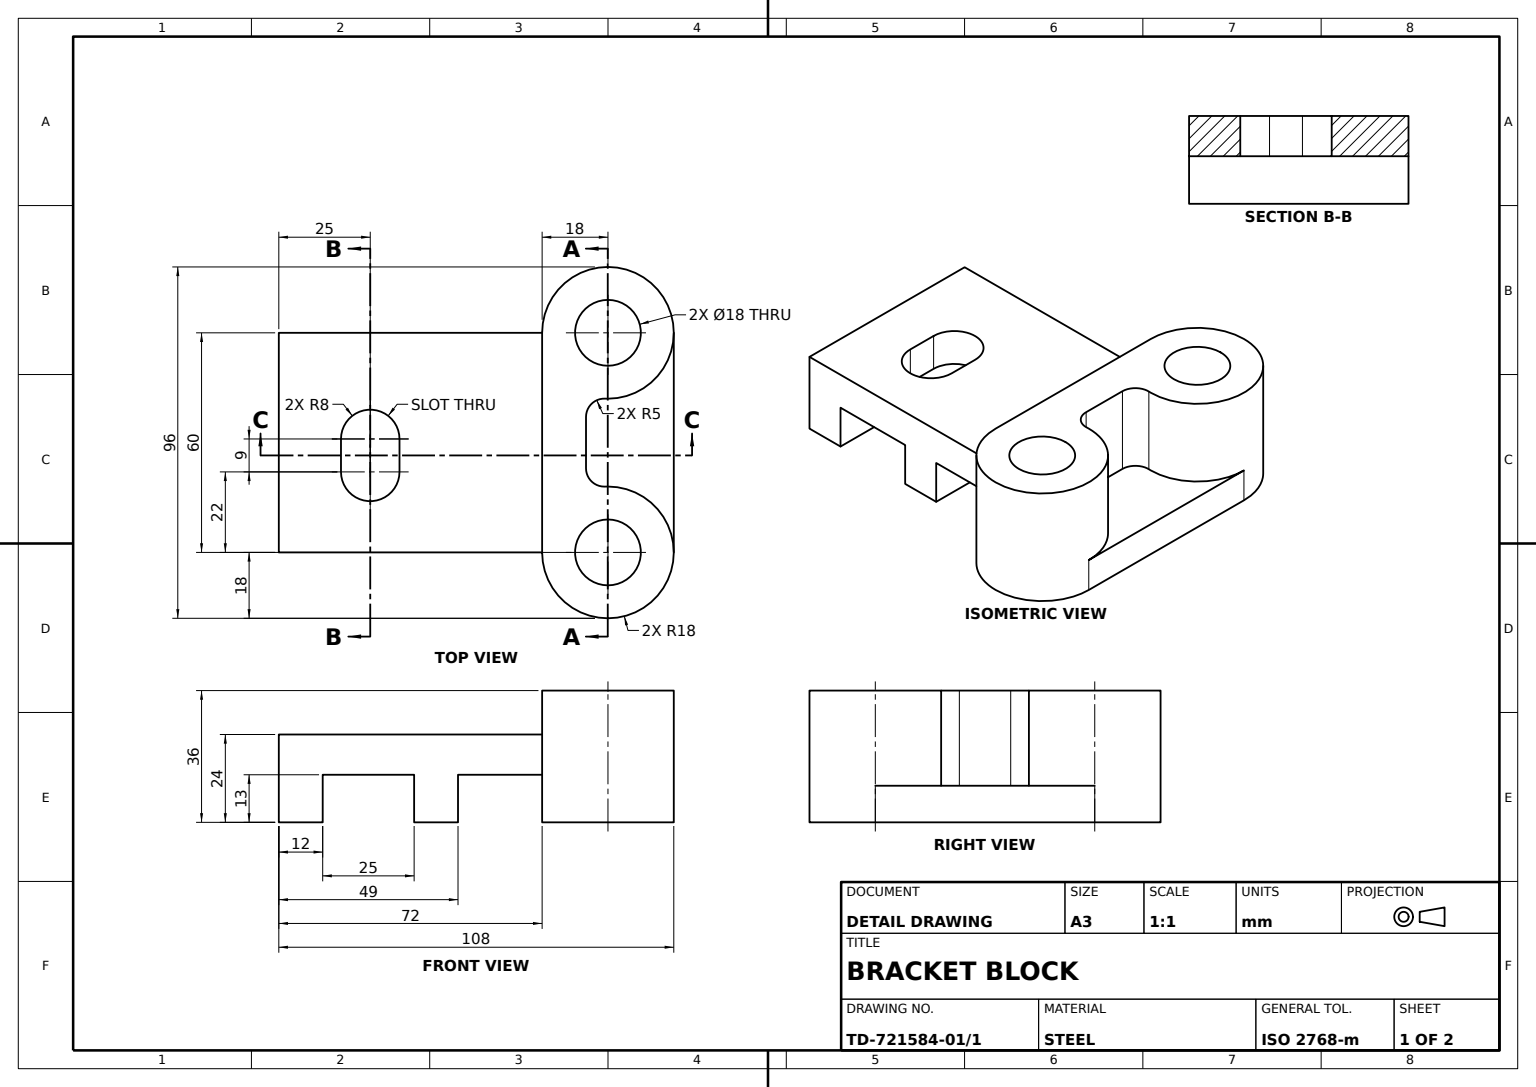
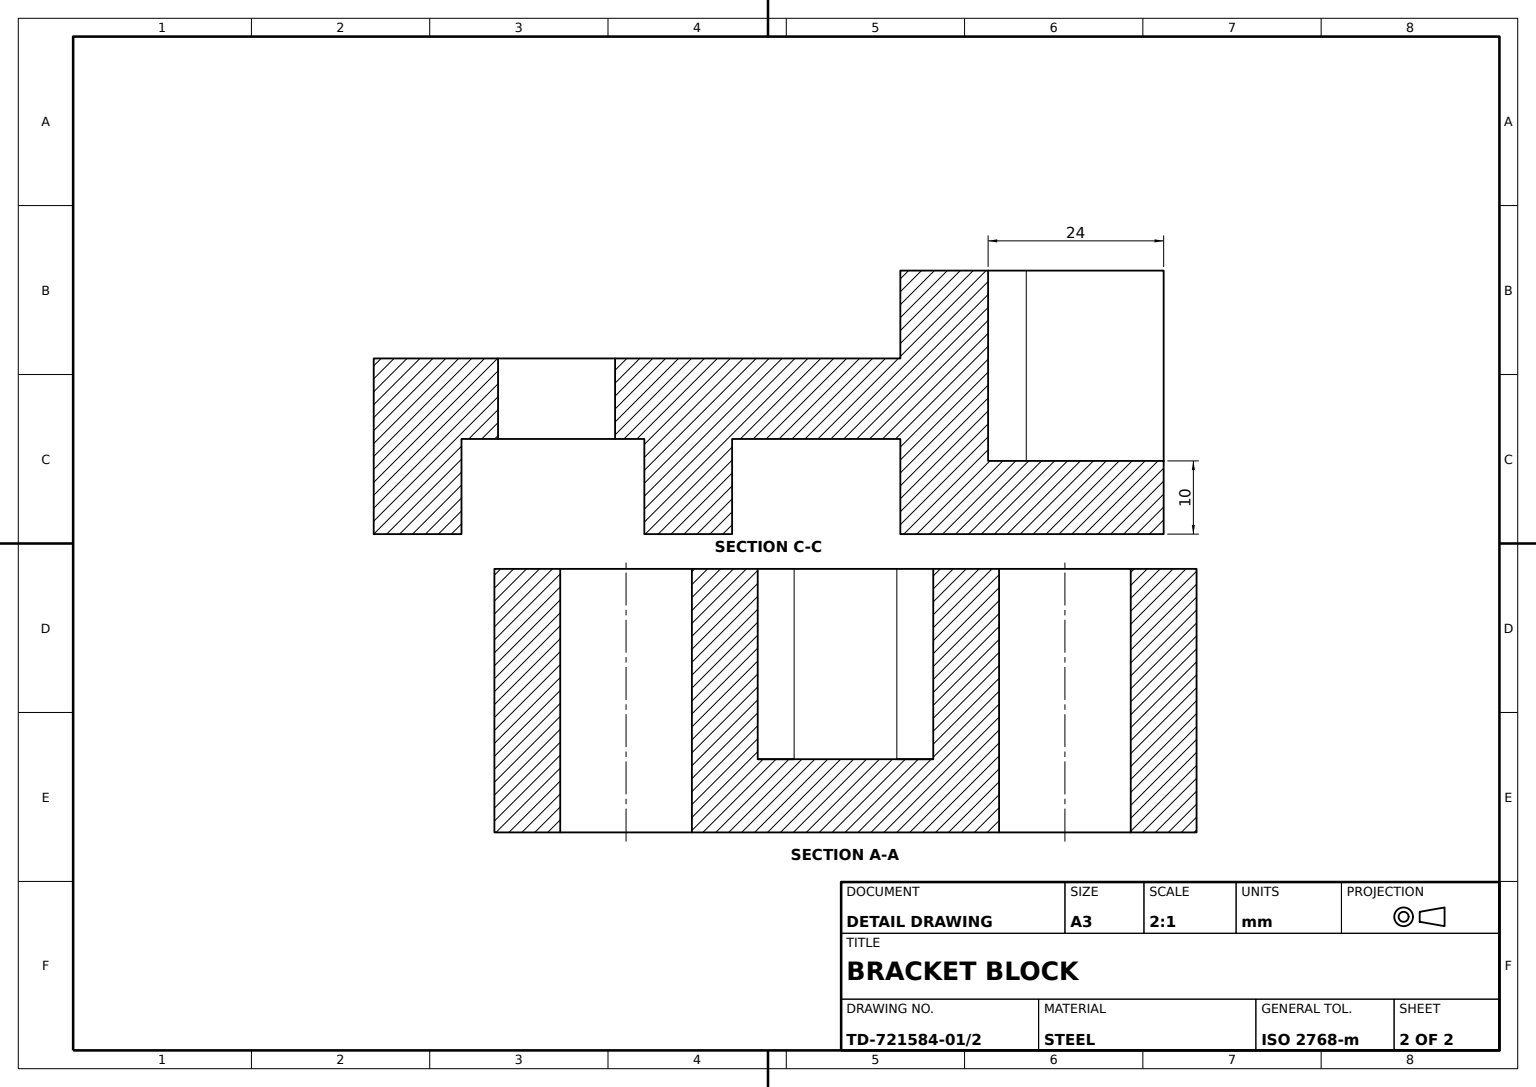
ISO-10303-21;
HEADER;
FILE_DESCRIPTION((''),'2;1');
FILE_NAME('','',(''),(''),'','','');
FILE_SCHEMA(('AUTOMOTIVE_DESIGN'));
ENDSEC;
DATA;
#1=APPLICATION_CONTEXT('');
#2=PRODUCT_CONTEXT('',#1,'mechanical');
#3=PRODUCT('','','',(#2));
#4=PRODUCT_DEFINITION_FORMATION('','',#3);
#5=PRODUCT_DEFINITION_CONTEXT('',#1,'design');
#6=PRODUCT_DEFINITION('','',#4,#5);
#7=PRODUCT_DEFINITION_SHAPE('','',#6);
#8=(LENGTH_UNIT()NAMED_UNIT(*)SI_UNIT(.MILLI.,.METRE.));
#9=(NAMED_UNIT(*)PLANE_ANGLE_UNIT()SI_UNIT($,.RADIAN.));
#10=(NAMED_UNIT(*)SI_UNIT($,.STERADIAN.)SOLID_ANGLE_UNIT());
#11=UNCERTAINTY_MEASURE_WITH_UNIT(LENGTH_MEASURE(1.E-05),#8,'distance_accuracy_value','');
#12=(GEOMETRIC_REPRESENTATION_CONTEXT(3)GLOBAL_UNCERTAINTY_ASSIGNED_CONTEXT((#11))GLOBAL_UNIT_ASSIGNED_CONTEXT((#8,#9,#10))REPRESENTATION_CONTEXT('',''));
#13=CARTESIAN_POINT('',(84.,10.,22.978251));
#14=VERTEX_POINT('',#13);
#15=CARTESIAN_POINT('',(89.217391,10.,17.982979));
#16=VERTEX_POINT('',#15);
#17=CARTESIAN_POINT('',(89.,10.,22.978251));
#18=DIRECTION('',(0.,-1.,0.));
#19=DIRECTION('',(0.,0.,1.));
#20=AXIS2_PLACEMENT_3D('',#17,#18,#19);
#21=CIRCLE('',#20,5.);
#22=EDGE_CURVE('',#14,#16,#21,.T.);
#23=ORIENTED_EDGE('',*,*,#22,.T.);
#24=CARTESIAN_POINT('',(89.217391,36.,17.982979));
#25=VERTEX_POINT('',#24);
#26=CARTESIAN_POINT('',(89.217391,0.,17.982979));
#27=DIRECTION('',(0.,1.,0.));
#28=VECTOR('',#27,1000.);
#29=LINE('',#26,#28);
#30=EDGE_CURVE('',#16,#25,#29,.T.);
#31=ORIENTED_EDGE('',*,*,#30,.T.);
#32=CARTESIAN_POINT('',(84.,36.,22.978251));
#33=VERTEX_POINT('',#32);
#34=CARTESIAN_POINT('',(89.,36.,22.978251));
#35=AXIS2_PLACEMENT_3D('',#34,#18,#19);
#36=CIRCLE('',#35,5.);
#37=EDGE_CURVE('',#33,#25,#36,.T.);
#38=ORIENTED_EDGE('',*,*,#37,.F.);
#39=CARTESIAN_POINT('',(84.,0.,22.978251));
#40=LINE('',#39,#28);
#41=EDGE_CURVE('',#14,#33,#40,.T.);
#42=ORIENTED_EDGE('',*,*,#41,.F.);
#43=EDGE_LOOP('',(#23,#31,#38,#42));
#44=FACE_OUTER_BOUND('',#43,.T.);
#45=CARTESIAN_POINT('',(89.,0.,22.978251));
#46=AXIS2_PLACEMENT_3D('',#45,#27,#19);
#47=CYLINDRICAL_SURFACE('',#46,5.);
#48=ADVANCED_FACE('',(#44),#47,.F.);
#49=CARTESIAN_POINT('',(33.,24.,29.));
#50=VERTEX_POINT('',#49);
#51=CARTESIAN_POINT('',(17.,24.,29.));
#52=VERTEX_POINT('',#51);
#53=CARTESIAN_POINT('',(25.,24.,29.));
#54=DIRECTION('',(-1.,0.,0.));
#55=AXIS2_PLACEMENT_3D('',#53,#27,#54);
#56=CIRCLE('',#55,8.);
#57=EDGE_CURVE('',#50,#52,#56,.T.);
#58=ORIENTED_EDGE('',*,*,#57,.F.);
#59=CARTESIAN_POINT('',(33.,24.,38.));
#60=VERTEX_POINT('',#59);
#61=DIRECTION('',(0.,0.,-1.));
#62=VECTOR('',#61,1000.);
#63=LINE('',#49,#62);
#64=EDGE_CURVE('',#60,#50,#63,.T.);
#65=ORIENTED_EDGE('',*,*,#64,.F.);
#66=CARTESIAN_POINT('',(17.,24.,38.));
#67=VERTEX_POINT('',#66);
#68=CARTESIAN_POINT('',(25.,24.,38.));
#69=AXIS2_PLACEMENT_3D('',#68,#27,#54);
#70=CIRCLE('',#69,8.);
#71=EDGE_CURVE('',#67,#60,#70,.T.);
#72=ORIENTED_EDGE('',*,*,#71,.F.);
#73=VECTOR('',#19,1000.);
#74=LINE('',#51,#73);
#75=EDGE_CURVE('',#52,#67,#74,.T.);
#76=ORIENTED_EDGE('',*,*,#75,.F.);
#77=EDGE_LOOP('',(#58,#65,#72,#76));
#78=FACE_BOUND('',#77,.T.);
#79=CARTESIAN_POINT('',(72.,24.,0.));
#80=VERTEX_POINT('',#79);
#81=CARTESIAN_POINT('',(0.,24.,0.));
#82=VERTEX_POINT('',#81);
#83=VECTOR('',#54,1000.);
#84=LINE('',#79,#83);
#85=EDGE_CURVE('',#80,#82,#84,.T.);
#86=ORIENTED_EDGE('',*,*,#85,.T.);
#87=CARTESIAN_POINT('',(0.,24.,60.));
#88=VERTEX_POINT('',#87);
#89=LINE('',#87,#62);
#90=EDGE_CURVE('',#88,#82,#89,.T.);
#91=ORIENTED_EDGE('',*,*,#90,.F.);
#92=CARTESIAN_POINT('',(72.,24.,60.));
#93=VERTEX_POINT('',#92);
#94=LINE('',#92,#83);
#95=EDGE_CURVE('',#93,#88,#94,.T.);
#96=ORIENTED_EDGE('',*,*,#95,.F.);
#97=LINE('',#92,#62);
#98=EDGE_CURVE('',#93,#80,#97,.T.);
#99=ORIENTED_EDGE('',*,*,#98,.T.);
#100=EDGE_LOOP('',(#86,#91,#96,#99));
#101=FACE_OUTER_BOUND('',#100,.T.);
#102=DIRECTION('',(1.,0.,0.));
#103=AXIS2_PLACEMENT_3D('',#92,#18,#102);
#104=PLANE('',#103);
#105=ADVANCED_FACE('',(#78,#101),#104,.F.);
#106=CARTESIAN_POINT('',(90.,0.,51.));
#107=VERTEX_POINT('',#106);
#108=CARTESIAN_POINT('',(90.,0.,69.));
#109=VERTEX_POINT('',#108);
#110=CARTESIAN_POINT('',(90.,0.,60.));
#111=AXIS2_PLACEMENT_3D('',#110,#27,#19);
#112=CIRCLE('',#111,9.);
#113=EDGE_CURVE('',#107,#109,#112,.T.);
#114=ORIENTED_EDGE('',*,*,#113,.F.);
#115=CARTESIAN_POINT('',(90.,36.,51.));
#116=VERTEX_POINT('',#115);
#117=LINE('',#106,#28);
#118=EDGE_CURVE('',#107,#116,#117,.T.);
#119=ORIENTED_EDGE('',*,*,#118,.T.);
#120=CARTESIAN_POINT('',(90.,36.,69.));
#121=VERTEX_POINT('',#120);
#122=CARTESIAN_POINT('',(90.,36.,60.));
#123=AXIS2_PLACEMENT_3D('',#122,#27,#19);
#124=CIRCLE('',#123,9.);
#125=EDGE_CURVE('',#116,#121,#124,.T.);
#126=ORIENTED_EDGE('',*,*,#125,.T.);
#127=LINE('',#108,#28);
#128=EDGE_CURVE('',#109,#121,#127,.T.);
#129=ORIENTED_EDGE('',*,*,#128,.F.);
#130=EDGE_LOOP('',(#114,#119,#126,#129));
#131=FACE_OUTER_BOUND('',#130,.T.);
#132=CYLINDRICAL_SURFACE('',#111,9.);
#133=ADVANCED_FACE('',(#131),#132,.F.);
#134=CARTESIAN_POINT('',(90.,0.,-9.));
#135=VERTEX_POINT('',#134);
#136=CARTESIAN_POINT('',(90.,0.,9.));
#137=VERTEX_POINT('',#136);
#138=CARTESIAN_POINT('',(90.,0.,0.));
#139=AXIS2_PLACEMENT_3D('',#138,#27,#19);
#140=CIRCLE('',#139,9.);
#141=EDGE_CURVE('',#135,#137,#140,.T.);
#142=ORIENTED_EDGE('',*,*,#141,.T.);
#143=EDGE_CURVE('',#137,#135,#140,.T.);
#144=ORIENTED_EDGE('',*,*,#143,.T.);
#145=EDGE_LOOP('',(#142,#144));
#146=FACE_BOUND('',#145,.T.);
#147=ORIENTED_EDGE('',*,*,#113,.T.);
#148=EDGE_CURVE('',#109,#107,#112,.T.);
#149=ORIENTED_EDGE('',*,*,#148,.T.);
#150=EDGE_LOOP('',(#147,#149));
#151=FACE_BOUND('',#150,.T.);
#152=CARTESIAN_POINT('',(108.,0.,0.));
#153=VERTEX_POINT('',#152);
#154=CARTESIAN_POINT('',(108.,0.,60.));
#155=VERTEX_POINT('',#154);
#156=LINE('',#152,#73);
#157=EDGE_CURVE('',#153,#155,#156,.T.);
#158=ORIENTED_EDGE('',*,*,#157,.T.);
#159=CARTESIAN_POINT('',(90.,0.,78.));
#160=VERTEX_POINT('',#159);
#161=CIRCLE('',#111,18.);
#162=EDGE_CURVE('',#160,#155,#161,.T.);
#163=ORIENTED_EDGE('',*,*,#162,.F.);
#164=CARTESIAN_POINT('',(72.,0.,60.));
#165=VERTEX_POINT('',#164);
#166=EDGE_CURVE('',#165,#160,#161,.T.);
#167=ORIENTED_EDGE('',*,*,#166,.F.);
#168=CARTESIAN_POINT('',(72.,0.,0.));
#169=VERTEX_POINT('',#168);
#170=LINE('',#168,#73);
#171=EDGE_CURVE('',#169,#165,#170,.T.);
#172=ORIENTED_EDGE('',*,*,#171,.F.);
#173=CARTESIAN_POINT('',(90.,0.,-18.));
#174=VERTEX_POINT('',#173);
#175=CIRCLE('',#139,18.);
#176=EDGE_CURVE('',#174,#169,#175,.T.);
#177=ORIENTED_EDGE('',*,*,#176,.F.);
#178=EDGE_CURVE('',#153,#174,#175,.T.);
#179=ORIENTED_EDGE('',*,*,#178,.F.);
#180=EDGE_LOOP('',(#158,#163,#167,#172,#177,#179));
#181=FACE_OUTER_BOUND('',#180,.T.);
#182=PLANE('',#139);
#183=ADVANCED_FACE('',(#146,#151,#181),#182,.F.);
#184=CARTESIAN_POINT('',(84.,10.,37.021749));
#185=VERTEX_POINT('',#184);
#186=CARTESIAN_POINT('',(84.,36.,37.021749));
#187=VERTEX_POINT('',#186);
#188=CARTESIAN_POINT('',(84.,0.,37.021749));
#189=LINE('',#188,#28);
#190=EDGE_CURVE('',#185,#187,#189,.T.);
#191=ORIENTED_EDGE('',*,*,#190,.T.);
#192=CARTESIAN_POINT('',(89.,36.,42.021749));
#193=VERTEX_POINT('',#192);
#194=CARTESIAN_POINT('',(89.,36.,37.021749));
#195=AXIS2_PLACEMENT_3D('',#194,#18,#19);
#196=CIRCLE('',#195,5.);
#197=EDGE_CURVE('',#193,#187,#196,.T.);
#198=ORIENTED_EDGE('',*,*,#197,.F.);
#199=CARTESIAN_POINT('',(89.,10.,42.021749));
#200=VERTEX_POINT('',#199);
#201=CARTESIAN_POINT('',(89.,0.,42.021749));
#202=LINE('',#201,#28);
#203=EDGE_CURVE('',#200,#193,#202,.T.);
#204=ORIENTED_EDGE('',*,*,#203,.F.);
#205=CARTESIAN_POINT('',(89.,10.,37.021749));
#206=AXIS2_PLACEMENT_3D('',#205,#27,#19);
#207=CIRCLE('',#206,5.);
#208=EDGE_CURVE('',#185,#200,#207,.T.);
#209=ORIENTED_EDGE('',*,*,#208,.F.);
#210=EDGE_LOOP('',(#191,#198,#204,#209));
#211=FACE_OUTER_BOUND('',#210,.T.);
#212=CARTESIAN_POINT('',(89.,0.,37.021749));
#213=AXIS2_PLACEMENT_3D('',#212,#27,#19);
#214=CYLINDRICAL_SURFACE('',#213,5.);
#215=ADVANCED_FACE('',(#211),#214,.F.);
#216=CARTESIAN_POINT('',(49.,0.,0.));
#217=VERTEX_POINT('',#216);
#218=CARTESIAN_POINT('',(49.,13.,0.));
#219=VERTEX_POINT('',#218);
#220=LINE('',#216,#28);
#221=EDGE_CURVE('',#217,#219,#220,.T.);
#222=ORIENTED_EDGE('',*,*,#221,.T.);
#223=CARTESIAN_POINT('',(49.,13.,60.));
#224=VERTEX_POINT('',#223);
#225=LINE('',#223,#62);
#226=EDGE_CURVE('',#224,#219,#225,.T.);
#227=ORIENTED_EDGE('',*,*,#226,.F.);
#228=CARTESIAN_POINT('',(49.,0.,60.));
#229=VERTEX_POINT('',#228);
#230=LINE('',#228,#28);
#231=EDGE_CURVE('',#229,#224,#230,.T.);
#232=ORIENTED_EDGE('',*,*,#231,.F.);
#233=LINE('',#228,#62);
#234=EDGE_CURVE('',#229,#217,#233,.T.);
#235=ORIENTED_EDGE('',*,*,#234,.T.);
#236=EDGE_LOOP('',(#222,#227,#232,#235));
#237=FACE_OUTER_BOUND('',#236,.T.);
#238=AXIS2_PLACEMENT_3D('',#228,#54,#19);
#239=PLANE('',#238);
#240=ADVANCED_FACE('',(#237),#239,.F.);
#241=CARTESIAN_POINT('',(108.,10.,0.));
#242=VERTEX_POINT('',#241);
#243=VECTOR('',#18,1000.);
#244=LINE('',#241,#243);
#245=EDGE_CURVE('',#242,#153,#244,.T.);
#246=ORIENTED_EDGE('',*,*,#245,.F.);
#247=CARTESIAN_POINT('',(108.,10.,60.));
#248=VERTEX_POINT('',#247);
#249=LINE('',#241,#73);
#250=EDGE_CURVE('',#242,#248,#249,.T.);
#251=ORIENTED_EDGE('',*,*,#250,.T.);
#252=LINE('',#247,#243);
#253=EDGE_CURVE('',#248,#155,#252,.T.);
#254=ORIENTED_EDGE('',*,*,#253,.T.);
#255=ORIENTED_EDGE('',*,*,#157,.F.);
#256=EDGE_LOOP('',(#246,#251,#254,#255));
#257=FACE_OUTER_BOUND('',#256,.T.);
#258=AXIS2_PLACEMENT_3D('',#241,#102,#61);
#259=PLANE('',#258);
#260=ADVANCED_FACE('',(#257),#259,.T.);
#261=CARTESIAN_POINT('',(90.,10.,18.));
#262=VERTEX_POINT('',#261);
#263=CARTESIAN_POINT('',(90.,36.,18.));
#264=VERTEX_POINT('',#263);
#265=CARTESIAN_POINT('',(90.,0.,18.));
#266=LINE('',#265,#28);
#267=EDGE_CURVE('',#262,#264,#266,.T.);
#268=ORIENTED_EDGE('',*,*,#267,.F.);
#269=CARTESIAN_POINT('',(90.,10.,0.));
#270=AXIS2_PLACEMENT_3D('',#269,#27,#19);
#271=CIRCLE('',#270,18.);
#272=EDGE_CURVE('',#262,#242,#271,.T.);
#273=ORIENTED_EDGE('',*,*,#272,.T.);
#274=ORIENTED_EDGE('',*,*,#245,.T.);
#275=ORIENTED_EDGE('',*,*,#178,.T.);
#276=CARTESIAN_POINT('',(90.,36.,-18.));
#277=VERTEX_POINT('',#276);
#278=LINE('',#173,#28);
#279=EDGE_CURVE('',#174,#277,#278,.T.);
#280=ORIENTED_EDGE('',*,*,#279,.T.);
#281=CARTESIAN_POINT('',(90.,36.,0.));
#282=AXIS2_PLACEMENT_3D('',#281,#27,#19);
#283=CIRCLE('',#282,18.);
#284=EDGE_CURVE('',#264,#277,#283,.T.);
#285=ORIENTED_EDGE('',*,*,#284,.F.);
#286=EDGE_LOOP('',(#268,#273,#274,#275,#280,#285));
#287=FACE_OUTER_BOUND('',#286,.T.);
#288=CYLINDRICAL_SURFACE('',#139,18.);
#289=ADVANCED_FACE('',(#287),#288,.T.);
#290=CARTESIAN_POINT('',(90.,10.,42.));
#291=VERTEX_POINT('',#290);
#292=CARTESIAN_POINT('',(89.217391,10.,42.017021));
#293=VERTEX_POINT('',#292);
#294=CARTESIAN_POINT('',(90.,10.,60.));
#295=AXIS2_PLACEMENT_3D('',#294,#27,#19);
#296=CIRCLE('',#295,18.);
#297=EDGE_CURVE('',#291,#293,#296,.T.);
#298=ORIENTED_EDGE('',*,*,#297,.T.);
#299=CARTESIAN_POINT('',(89.217391,36.,42.017021));
#300=VERTEX_POINT('',#299);
#301=CARTESIAN_POINT('',(89.217391,0.,42.017021));
#302=LINE('',#301,#28);
#303=EDGE_CURVE('',#293,#300,#302,.T.);
#304=ORIENTED_EDGE('',*,*,#303,.T.);
#305=CARTESIAN_POINT('',(90.,36.,42.));
#306=VERTEX_POINT('',#305);
#307=CIRCLE('',#123,18.);
#308=EDGE_CURVE('',#306,#300,#307,.T.);
#309=ORIENTED_EDGE('',*,*,#308,.F.);
#310=CARTESIAN_POINT('',(90.,0.,42.));
#311=LINE('',#310,#28);
#312=EDGE_CURVE('',#291,#306,#311,.T.);
#313=ORIENTED_EDGE('',*,*,#312,.F.);
#314=EDGE_LOOP('',(#298,#304,#309,#313));
#315=FACE_OUTER_BOUND('',#314,.T.);
#316=CYLINDRICAL_SURFACE('',#111,18.);
#317=ADVANCED_FACE('',(#315),#316,.T.);
#318=ORIENTED_EDGE('',*,*,#226,.T.);
#319=CARTESIAN_POINT('',(72.,13.,0.));
#320=VERTEX_POINT('',#319);
#321=VECTOR('',#102,1000.);
#322=LINE('',#218,#321);
#323=EDGE_CURVE('',#219,#320,#322,.T.);
#324=ORIENTED_EDGE('',*,*,#323,.T.);
#325=CARTESIAN_POINT('',(72.,13.,60.));
#326=VERTEX_POINT('',#325);
#327=LINE('',#325,#62);
#328=EDGE_CURVE('',#326,#320,#327,.T.);
#329=ORIENTED_EDGE('',*,*,#328,.F.);
#330=LINE('',#223,#321);
#331=EDGE_CURVE('',#224,#326,#330,.T.);
#332=ORIENTED_EDGE('',*,*,#331,.F.);
#333=EDGE_LOOP('',(#318,#324,#329,#332));
#334=FACE_OUTER_BOUND('',#333,.T.);
#335=AXIS2_PLACEMENT_3D('',#223,#27,#19);
#336=PLANE('',#335);
#337=ADVANCED_FACE('',(#334),#336,.F.);
#338=CARTESIAN_POINT('',(33.,13.,38.));
#339=VERTEX_POINT('',#338);
#340=CARTESIAN_POINT('',(33.,13.,29.));
#341=VERTEX_POINT('',#340);
#342=CARTESIAN_POINT('',(33.,13.,60.));
#343=LINE('',#342,#62);
#344=EDGE_CURVE('',#339,#341,#343,.T.);
#345=ORIENTED_EDGE('',*,*,#344,.F.);
#346=CARTESIAN_POINT('',(33.,0.,38.));
#347=LINE('',#346,#28);
#348=EDGE_CURVE('',#339,#60,#347,.T.);
#349=ORIENTED_EDGE('',*,*,#348,.T.);
#350=ORIENTED_EDGE('',*,*,#64,.T.);
#351=CARTESIAN_POINT('',(33.,0.,29.));
#352=LINE('',#351,#28);
#353=EDGE_CURVE('',#341,#50,#352,.T.);
#354=ORIENTED_EDGE('',*,*,#353,.F.);
#355=EDGE_LOOP('',(#345,#349,#350,#354));
#356=FACE_OUTER_BOUND('',#355,.T.);
#357=AXIS2_PLACEMENT_3D('',#351,#102,#61);
#358=PLANE('',#357);
#359=ADVANCED_FACE('',(#356),#358,.F.);
#360=EDGE_CURVE('',#121,#116,#124,.T.);
#361=ORIENTED_EDGE('',*,*,#360,.T.);
#362=ORIENTED_EDGE('',*,*,#118,.F.);
#363=ORIENTED_EDGE('',*,*,#148,.F.);
#364=ORIENTED_EDGE('',*,*,#128,.T.);
#365=EDGE_LOOP('',(#361,#362,#363,#364));
#366=FACE_OUTER_BOUND('',#365,.T.);
#367=ADVANCED_FACE('',(#366),#132,.F.);
#368=ORIENTED_EDGE('',*,*,#279,.F.);
#369=ORIENTED_EDGE('',*,*,#176,.T.);
#370=LINE('',#168,#28);
#371=EDGE_CURVE('',#169,#320,#370,.T.);
#372=ORIENTED_EDGE('',*,*,#371,.T.);
#373=LINE('',#319,#28);
#374=EDGE_CURVE('',#320,#80,#373,.T.);
#375=ORIENTED_EDGE('',*,*,#374,.T.);
#376=CARTESIAN_POINT('',(72.,36.,0.));
#377=VERTEX_POINT('',#376);
#378=EDGE_CURVE('',#80,#377,#370,.T.);
#379=ORIENTED_EDGE('',*,*,#378,.T.);
#380=EDGE_CURVE('',#277,#377,#283,.T.);
#381=ORIENTED_EDGE('',*,*,#380,.F.);
#382=EDGE_LOOP('',(#368,#369,#372,#375,#379,#381));
#383=FACE_OUTER_BOUND('',#382,.T.);
#384=ADVANCED_FACE('',(#383),#288,.T.);
#385=ORIENTED_EDGE('',*,*,#57,.T.);
#386=CARTESIAN_POINT('',(17.,13.,29.));
#387=VERTEX_POINT('',#386);
#388=CARTESIAN_POINT('',(17.,0.,29.));
#389=LINE('',#388,#28);
#390=EDGE_CURVE('',#387,#52,#389,.T.);
#391=ORIENTED_EDGE('',*,*,#390,.F.);
#392=CARTESIAN_POINT('',(25.,13.,29.));
#393=AXIS2_PLACEMENT_3D('',#392,#27,#19);
#394=CIRCLE('',#393,8.);
#395=EDGE_CURVE('',#341,#387,#394,.T.);
#396=ORIENTED_EDGE('',*,*,#395,.F.);
#397=ORIENTED_EDGE('',*,*,#353,.T.);
#398=EDGE_LOOP('',(#385,#391,#396,#397));
#399=FACE_OUTER_BOUND('',#398,.T.);
#400=CARTESIAN_POINT('',(25.,0.,29.));
#401=AXIS2_PLACEMENT_3D('',#400,#27,#54);
#402=CYLINDRICAL_SURFACE('',#401,8.);
#403=ADVANCED_FACE('',(#399),#402,.F.);
#404=CARTESIAN_POINT('',(72.,36.,60.));
#405=VERTEX_POINT('',#404);
#406=LINE('',#376,#73);
#407=EDGE_CURVE('',#377,#405,#406,.T.);
#408=ORIENTED_EDGE('',*,*,#407,.F.);
#409=ORIENTED_EDGE('',*,*,#378,.F.);
#410=ORIENTED_EDGE('',*,*,#98,.F.);
#411=LINE('',#164,#28);
#412=EDGE_CURVE('',#93,#405,#411,.T.);
#413=ORIENTED_EDGE('',*,*,#412,.T.);
#414=EDGE_LOOP('',(#408,#409,#410,#413));
#415=FACE_OUTER_BOUND('',#414,.T.);
#416=AXIS2_PLACEMENT_3D('',#168,#54,#19);
#417=PLANE('',#416);
#418=ADVANCED_FACE('',(#415),#417,.T.);
#419=LINE('',#32,#62);
#420=EDGE_CURVE('',#187,#33,#419,.T.);
#421=ORIENTED_EDGE('',*,*,#420,.F.);
#422=ORIENTED_EDGE('',*,*,#190,.F.);
#423=CARTESIAN_POINT('',(84.,10.,0.));
#424=LINE('',#423,#73);
#425=EDGE_CURVE('',#14,#185,#424,.T.);
#426=ORIENTED_EDGE('',*,*,#425,.F.);
#427=ORIENTED_EDGE('',*,*,#41,.T.);
#428=EDGE_LOOP('',(#421,#422,#426,#427));
#429=FACE_OUTER_BOUND('',#428,.T.);
#430=AXIS2_PLACEMENT_3D('',#39,#102,#61);
#431=PLANE('',#430);
#432=ADVANCED_FACE('',(#429),#431,.T.);
#433=ORIENTED_EDGE('',*,*,#37,.T.);
#434=EDGE_CURVE('',#25,#264,#283,.T.);
#435=ORIENTED_EDGE('',*,*,#434,.T.);
#436=ORIENTED_EDGE('',*,*,#284,.T.);
#437=ORIENTED_EDGE('',*,*,#380,.T.);
#438=ORIENTED_EDGE('',*,*,#407,.T.);
#439=CARTESIAN_POINT('',(90.,36.,78.));
#440=VERTEX_POINT('',#439);
#441=EDGE_CURVE('',#405,#440,#307,.T.);
#442=ORIENTED_EDGE('',*,*,#441,.T.);
#443=EDGE_CURVE('',#440,#306,#307,.T.);
#444=ORIENTED_EDGE('',*,*,#443,.T.);
#445=ORIENTED_EDGE('',*,*,#308,.T.);
#446=EDGE_CURVE('',#300,#193,#196,.T.);
#447=ORIENTED_EDGE('',*,*,#446,.T.);
#448=ORIENTED_EDGE('',*,*,#197,.T.);
#449=ORIENTED_EDGE('',*,*,#420,.T.);
#450=EDGE_LOOP('',(#433,#435,#436,#437,#438,#442,#444,#445,#447,#448,#449));
#451=FACE_OUTER_BOUND('',#450,.T.);
#452=ORIENTED_EDGE('',*,*,#360,.F.);
#453=ORIENTED_EDGE('',*,*,#125,.F.);
#454=EDGE_LOOP('',(#452,#453));
#455=FACE_BOUND('',#454,.T.);
#456=CARTESIAN_POINT('',(90.,36.,9.));
#457=VERTEX_POINT('',#456);
#458=CARTESIAN_POINT('',(90.,36.,-9.));
#459=VERTEX_POINT('',#458);
#460=CIRCLE('',#282,9.);
#461=EDGE_CURVE('',#457,#459,#460,.T.);
#462=ORIENTED_EDGE('',*,*,#461,.F.);
#463=EDGE_CURVE('',#459,#457,#460,.T.);
#464=ORIENTED_EDGE('',*,*,#463,.F.);
#465=EDGE_LOOP('',(#462,#464));
#466=FACE_BOUND('',#465,.T.);
#467=PLANE('',#282);
#468=ADVANCED_FACE('',(#451,#455,#466),#467,.T.);
#469=CARTESIAN_POINT('',(0.,0.,60.));
#470=VERTEX_POINT('',#469);
#471=CARTESIAN_POINT('',(0.,0.,0.));
#472=VERTEX_POINT('',#471);
#473=LINE('',#469,#62);
#474=EDGE_CURVE('',#470,#472,#473,.T.);
#475=ORIENTED_EDGE('',*,*,#474,.T.);
#476=CARTESIAN_POINT('',(12.,0.,0.));
#477=VERTEX_POINT('',#476);
#478=LINE('',#471,#321);
#479=EDGE_CURVE('',#472,#477,#478,.T.);
#480=ORIENTED_EDGE('',*,*,#479,.T.);
#481=CARTESIAN_POINT('',(12.,0.,60.));
#482=VERTEX_POINT('',#481);
#483=LINE('',#481,#62);
#484=EDGE_CURVE('',#482,#477,#483,.T.);
#485=ORIENTED_EDGE('',*,*,#484,.F.);
#486=LINE('',#469,#321);
#487=EDGE_CURVE('',#470,#482,#486,.T.);
#488=ORIENTED_EDGE('',*,*,#487,.F.);
#489=EDGE_LOOP('',(#475,#480,#485,#488));
#490=FACE_OUTER_BOUND('',#489,.T.);
#491=AXIS2_PLACEMENT_3D('',#469,#27,#19);
#492=PLANE('',#491);
#493=ADVANCED_FACE('',(#490),#492,.F.);
#494=CARTESIAN_POINT('',(12.,13.,60.));
#495=VERTEX_POINT('',#494);
#496=CARTESIAN_POINT('',(37.,13.,60.));
#497=VERTEX_POINT('',#496);
#498=LINE('',#494,#321);
#499=EDGE_CURVE('',#495,#497,#498,.T.);
#500=ORIENTED_EDGE('',*,*,#499,.T.);
#501=CARTESIAN_POINT('',(37.,0.,60.));
#502=VERTEX_POINT('',#501);
#503=LINE('',#496,#243);
#504=EDGE_CURVE('',#497,#502,#503,.T.);
#505=ORIENTED_EDGE('',*,*,#504,.T.);
#506=LINE('',#501,#321);
#507=EDGE_CURVE('',#502,#229,#506,.T.);
#508=ORIENTED_EDGE('',*,*,#507,.T.);
#509=ORIENTED_EDGE('',*,*,#231,.T.);
#510=ORIENTED_EDGE('',*,*,#331,.T.);
#511=LINE('',#325,#28);
#512=EDGE_CURVE('',#326,#93,#511,.T.);
#513=ORIENTED_EDGE('',*,*,#512,.T.);
#514=ORIENTED_EDGE('',*,*,#95,.T.);
#515=LINE('',#87,#243);
#516=EDGE_CURVE('',#88,#470,#515,.T.);
#517=ORIENTED_EDGE('',*,*,#516,.T.);
#518=ORIENTED_EDGE('',*,*,#487,.T.);
#519=LINE('',#481,#28);
#520=EDGE_CURVE('',#482,#495,#519,.T.);
#521=ORIENTED_EDGE('',*,*,#520,.T.);
#522=EDGE_LOOP('',(#500,#505,#508,#509,#510,#513,#514,#517,#518,#521));
#523=FACE_OUTER_BOUND('',#522,.T.);
#524=AXIS2_PLACEMENT_3D('',#469,#19,#102);
#525=PLANE('',#524);
#526=ADVANCED_FACE('',(#523),#525,.T.);
#527=ORIENTED_EDGE('',*,*,#166,.T.);
#528=LINE('',#159,#28);
#529=EDGE_CURVE('',#160,#440,#528,.T.);
#530=ORIENTED_EDGE('',*,*,#529,.T.);
#531=ORIENTED_EDGE('',*,*,#441,.F.);
#532=ORIENTED_EDGE('',*,*,#412,.F.);
#533=ORIENTED_EDGE('',*,*,#512,.F.);
#534=EDGE_CURVE('',#165,#326,#411,.T.);
#535=ORIENTED_EDGE('',*,*,#534,.F.);
#536=EDGE_LOOP('',(#527,#530,#531,#532,#533,#535));
#537=FACE_OUTER_BOUND('',#536,.T.);
#538=ADVANCED_FACE('',(#537),#316,.T.);
#539=EDGE_CURVE('',#248,#291,#296,.T.);
#540=ORIENTED_EDGE('',*,*,#539,.T.);
#541=ORIENTED_EDGE('',*,*,#312,.T.);
#542=ORIENTED_EDGE('',*,*,#443,.F.);
#543=ORIENTED_EDGE('',*,*,#529,.F.);
#544=ORIENTED_EDGE('',*,*,#162,.T.);
#545=ORIENTED_EDGE('',*,*,#253,.F.);
#546=EDGE_LOOP('',(#540,#541,#542,#543,#544,#545));
#547=FACE_OUTER_BOUND('',#546,.T.);
#548=ADVANCED_FACE('',(#547),#316,.T.);
#549=ORIENTED_EDGE('',*,*,#507,.F.);
#550=CARTESIAN_POINT('',(37.,0.,0.));
#551=VERTEX_POINT('',#550);
#552=LINE('',#501,#62);
#553=EDGE_CURVE('',#502,#551,#552,.T.);
#554=ORIENTED_EDGE('',*,*,#553,.T.);
#555=LINE('',#550,#321);
#556=EDGE_CURVE('',#551,#217,#555,.T.);
#557=ORIENTED_EDGE('',*,*,#556,.T.);
#558=ORIENTED_EDGE('',*,*,#234,.F.);
#559=EDGE_LOOP('',(#549,#554,#557,#558));
#560=FACE_OUTER_BOUND('',#559,.T.);
#561=AXIS2_PLACEMENT_3D('',#501,#27,#19);
#562=PLANE('',#561);
#563=ADVANCED_FACE('',(#560),#562,.F.);
#564=ORIENTED_EDGE('',*,*,#484,.T.);
#565=CARTESIAN_POINT('',(12.,13.,0.));
#566=VERTEX_POINT('',#565);
#567=LINE('',#476,#28);
#568=EDGE_CURVE('',#477,#566,#567,.T.);
#569=ORIENTED_EDGE('',*,*,#568,.T.);
#570=LINE('',#494,#62);
#571=EDGE_CURVE('',#495,#566,#570,.T.);
#572=ORIENTED_EDGE('',*,*,#571,.F.);
#573=ORIENTED_EDGE('',*,*,#520,.F.);
#574=EDGE_LOOP('',(#564,#569,#572,#573));
#575=FACE_OUTER_BOUND('',#574,.T.);
#576=AXIS2_PLACEMENT_3D('',#481,#54,#19);
#577=PLANE('',#576);
#578=ADVANCED_FACE('',(#575),#577,.F.);
#579=ORIENTED_EDGE('',*,*,#71,.T.);
#580=ORIENTED_EDGE('',*,*,#348,.F.);
#581=CARTESIAN_POINT('',(17.,13.,38.));
#582=VERTEX_POINT('',#581);
#583=CARTESIAN_POINT('',(25.,13.,38.));
#584=AXIS2_PLACEMENT_3D('',#583,#27,#19);
#585=CIRCLE('',#584,8.);
#586=EDGE_CURVE('',#582,#339,#585,.T.);
#587=ORIENTED_EDGE('',*,*,#586,.F.);
#588=CARTESIAN_POINT('',(17.,0.,38.));
#589=LINE('',#588,#28);
#590=EDGE_CURVE('',#582,#67,#589,.T.);
#591=ORIENTED_EDGE('',*,*,#590,.T.);
#592=EDGE_LOOP('',(#579,#580,#587,#591));
#593=FACE_OUTER_BOUND('',#592,.T.);
#594=CARTESIAN_POINT('',(25.,0.,38.));
#595=AXIS2_PLACEMENT_3D('',#594,#27,#54);
#596=CYLINDRICAL_SURFACE('',#595,8.);
#597=ADVANCED_FACE('',(#593),#596,.F.);
#598=ORIENTED_EDGE('',*,*,#141,.F.);
#599=LINE('',#134,#28);
#600=EDGE_CURVE('',#135,#459,#599,.T.);
#601=ORIENTED_EDGE('',*,*,#600,.T.);
#602=ORIENTED_EDGE('',*,*,#463,.T.);
#603=LINE('',#136,#28);
#604=EDGE_CURVE('',#137,#457,#603,.T.);
#605=ORIENTED_EDGE('',*,*,#604,.F.);
#606=EDGE_LOOP('',(#598,#601,#602,#605));
#607=FACE_OUTER_BOUND('',#606,.T.);
#608=CYLINDRICAL_SURFACE('',#139,9.);
#609=ADVANCED_FACE('',(#607),#608,.F.);
#610=CARTESIAN_POINT('',(37.,13.,0.));
#611=VERTEX_POINT('',#610);
#612=LINE('',#565,#321);
#613=EDGE_CURVE('',#566,#611,#612,.T.);
#614=ORIENTED_EDGE('',*,*,#613,.F.);
#615=ORIENTED_EDGE('',*,*,#568,.F.);
#616=ORIENTED_EDGE('',*,*,#479,.F.);
#617=LINE('',#81,#243);
#618=EDGE_CURVE('',#82,#472,#617,.T.);
#619=ORIENTED_EDGE('',*,*,#618,.F.);
#620=ORIENTED_EDGE('',*,*,#85,.F.);
#621=ORIENTED_EDGE('',*,*,#374,.F.);
#622=ORIENTED_EDGE('',*,*,#323,.F.);
#623=ORIENTED_EDGE('',*,*,#221,.F.);
#624=ORIENTED_EDGE('',*,*,#556,.F.);
#625=LINE('',#610,#243);
#626=EDGE_CURVE('',#611,#551,#625,.T.);
#627=ORIENTED_EDGE('',*,*,#626,.F.);
#628=EDGE_LOOP('',(#614,#615,#616,#619,#620,#621,#622,#623,#624,#627));
#629=FACE_OUTER_BOUND('',#628,.T.);
#630=AXIS2_PLACEMENT_3D('',#471,#19,#102);
#631=PLANE('',#630);
#632=ADVANCED_FACE('',(#629),#631,.F.);
#633=ORIENTED_EDGE('',*,*,#395,.T.);
#634=CARTESIAN_POINT('',(17.,13.,60.));
#635=LINE('',#634,#73);
#636=EDGE_CURVE('',#387,#582,#635,.T.);
#637=ORIENTED_EDGE('',*,*,#636,.T.);
#638=ORIENTED_EDGE('',*,*,#586,.T.);
#639=ORIENTED_EDGE('',*,*,#344,.T.);
#640=EDGE_LOOP('',(#633,#637,#638,#639));
#641=FACE_BOUND('',#640,.T.);
#642=ORIENTED_EDGE('',*,*,#571,.T.);
#643=ORIENTED_EDGE('',*,*,#613,.T.);
#644=LINE('',#496,#62);
#645=EDGE_CURVE('',#497,#611,#644,.T.);
#646=ORIENTED_EDGE('',*,*,#645,.F.);
#647=ORIENTED_EDGE('',*,*,#499,.F.);
#648=EDGE_LOOP('',(#642,#643,#646,#647));
#649=FACE_OUTER_BOUND('',#648,.T.);
#650=AXIS2_PLACEMENT_3D('',#494,#27,#19);
#651=PLANE('',#650);
#652=ADVANCED_FACE('',(#641,#649),#651,.F.);
#653=ORIENTED_EDGE('',*,*,#90,.T.);
#654=ORIENTED_EDGE('',*,*,#618,.T.);
#655=ORIENTED_EDGE('',*,*,#474,.F.);
#656=ORIENTED_EDGE('',*,*,#516,.F.);
#657=EDGE_LOOP('',(#653,#654,#655,#656));
#658=FACE_OUTER_BOUND('',#657,.T.);
#659=AXIS2_PLACEMENT_3D('',#87,#102,#27);
#660=PLANE('',#659);
#661=ADVANCED_FACE('',(#658),#660,.F.);
#662=ORIENTED_EDGE('',*,*,#75,.T.);
#663=ORIENTED_EDGE('',*,*,#590,.F.);
#664=ORIENTED_EDGE('',*,*,#636,.F.);
#665=ORIENTED_EDGE('',*,*,#390,.T.);
#666=EDGE_LOOP('',(#662,#663,#664,#665));
#667=FACE_OUTER_BOUND('',#666,.T.);
#668=AXIS2_PLACEMENT_3D('',#388,#54,#19);
#669=PLANE('',#668);
#670=ADVANCED_FACE('',(#667),#669,.F.);
#671=ORIENTED_EDGE('',*,*,#645,.T.);
#672=ORIENTED_EDGE('',*,*,#626,.T.);
#673=ORIENTED_EDGE('',*,*,#553,.F.);
#674=ORIENTED_EDGE('',*,*,#504,.F.);
#675=EDGE_LOOP('',(#671,#672,#673,#674));
#676=FACE_OUTER_BOUND('',#675,.T.);
#677=AXIS2_PLACEMENT_3D('',#496,#102,#61);
#678=PLANE('',#677);
#679=ADVANCED_FACE('',(#676),#678,.F.);
#680=ORIENTED_EDGE('',*,*,#600,.F.);
#681=ORIENTED_EDGE('',*,*,#143,.F.);
#682=ORIENTED_EDGE('',*,*,#604,.T.);
#683=ORIENTED_EDGE('',*,*,#461,.T.);
#684=EDGE_LOOP('',(#680,#681,#682,#683));
#685=FACE_OUTER_BOUND('',#684,.T.);
#686=ADVANCED_FACE('',(#685),#608,.F.);
#687=ORIENTED_EDGE('',*,*,#371,.F.);
#688=ORIENTED_EDGE('',*,*,#171,.T.);
#689=ORIENTED_EDGE('',*,*,#534,.T.);
#690=ORIENTED_EDGE('',*,*,#328,.T.);
#691=EDGE_LOOP('',(#687,#688,#689,#690));
#692=FACE_OUTER_BOUND('',#691,.T.);
#693=ADVANCED_FACE('',(#692),#417,.T.);
#694=ORIENTED_EDGE('',*,*,#303,.F.);
#695=EDGE_CURVE('',#200,#293,#207,.T.);
#696=ORIENTED_EDGE('',*,*,#695,.F.);
#697=ORIENTED_EDGE('',*,*,#203,.T.);
#698=ORIENTED_EDGE('',*,*,#446,.F.);
#699=EDGE_LOOP('',(#694,#696,#697,#698));
#700=FACE_OUTER_BOUND('',#699,.T.);
#701=ADVANCED_FACE('',(#700),#214,.F.);
#702=ORIENTED_EDGE('',*,*,#272,.F.);
#703=EDGE_CURVE('',#16,#262,#271,.T.);
#704=ORIENTED_EDGE('',*,*,#703,.F.);
#705=ORIENTED_EDGE('',*,*,#22,.F.);
#706=ORIENTED_EDGE('',*,*,#425,.T.);
#707=ORIENTED_EDGE('',*,*,#208,.T.);
#708=ORIENTED_EDGE('',*,*,#695,.T.);
#709=ORIENTED_EDGE('',*,*,#297,.F.);
#710=ORIENTED_EDGE('',*,*,#539,.F.);
#711=ORIENTED_EDGE('',*,*,#250,.F.);
#712=EDGE_LOOP('',(#702,#704,#705,#706,#707,#708,#709,#710,#711));
#713=FACE_OUTER_BOUND('',#712,.T.);
#714=CARTESIAN_POINT('',(0.,10.,0.));
#715=AXIS2_PLACEMENT_3D('',#714,#27,#19);
#716=PLANE('',#715);
#717=ADVANCED_FACE('',(#713),#716,.T.);
#718=ORIENTED_EDGE('',*,*,#267,.T.);
#719=ORIENTED_EDGE('',*,*,#434,.F.);
#720=ORIENTED_EDGE('',*,*,#30,.F.);
#721=ORIENTED_EDGE('',*,*,#703,.T.);
#722=EDGE_LOOP('',(#718,#719,#720,#721));
#723=FACE_OUTER_BOUND('',#722,.T.);
#724=ADVANCED_FACE('',(#723),#288,.T.);
#725=CLOSED_SHELL('',(#48,#105,#133,#183,#215,#240,#260,#289,#317,#337,#359,#367,#384,#403,#418,#432,#468,#493,#526,#538,#548,#563,#578,#597,#609,#632,#652,#661,#670,#679,#686,#693,#701,#717,#724));
#726=MANIFOLD_SOLID_BREP('',#725);
#727=ADVANCED_BREP_SHAPE_REPRESENTATION('',(#726),#12);
#728=SHAPE_DEFINITION_REPRESENTATION(#7,#727);
ENDSEC;
END-ISO-10303-21;
